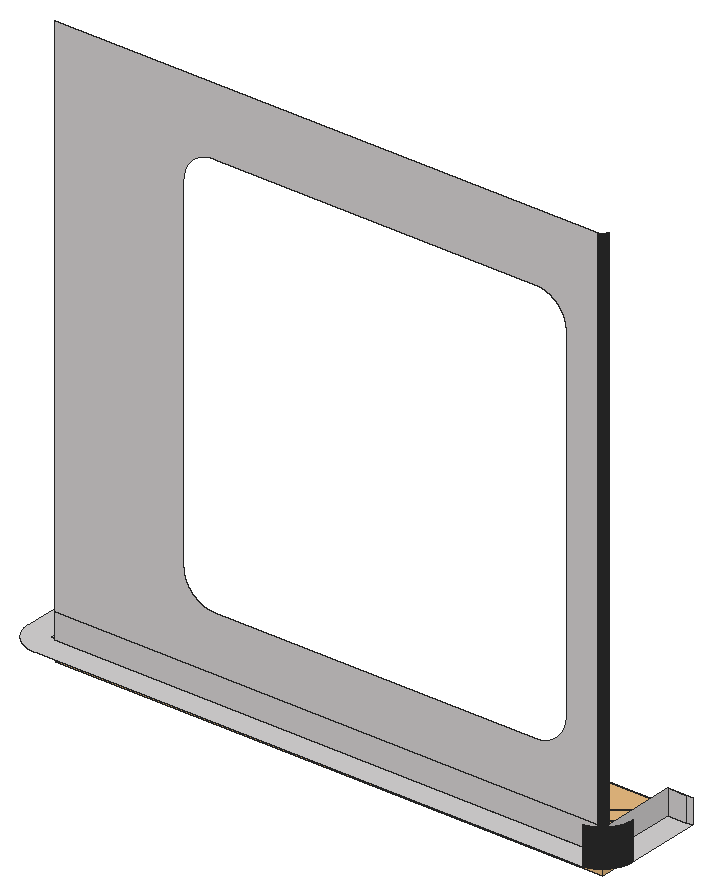
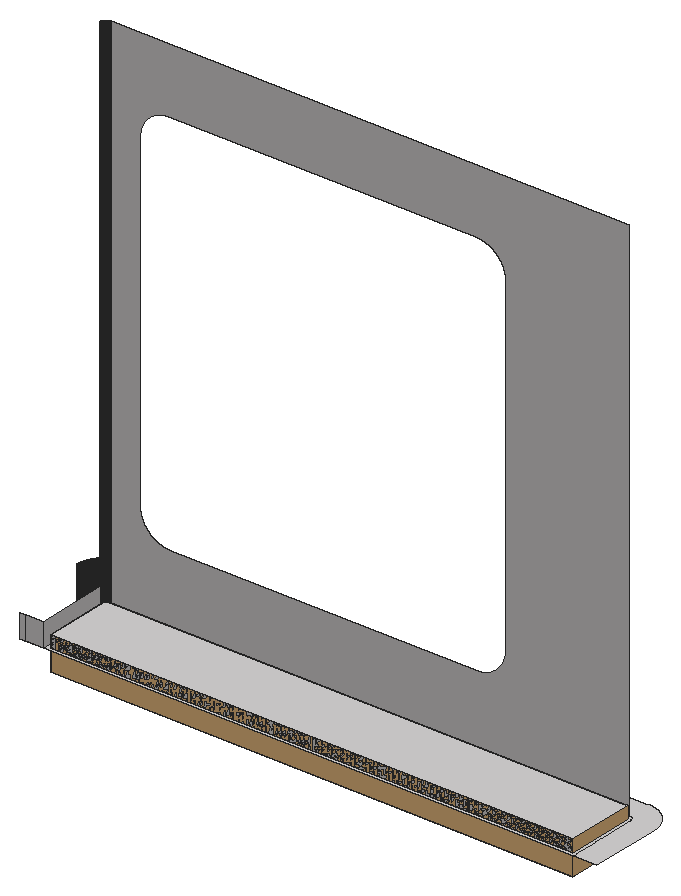
# SketchUp Ruby script. Lengths in inches.
U = 1.inch
M = Sketchup.active_model
def pt(a) = Geom::Point3d.new(a.map { |v| v * U })
def face(e, loops, mat)
  f = e.add_face(loops[0].map { |a| pt(a) })
  loops[1..].each { |l| e.add_face(l.map { |a| pt(a) }).erase! }
  f.material = f.back_material = mat if mat
  f
end
# faces: each face lists its corners as indices into pts; further lists are holes
def faces(e, pts, list, mat = nil) = list.each { |f| face(e, (f[0].is_a?(Array) ? f : [f]).map { |l| l.map { |i| pts[i] } }, mat) }
# xy, xz, yz: faces in a plane at the given z, y or x. An outline is a flat list of corners, or four numbers for a rectangle; further outlines are holes
def ring(l) = l.size == 4 ? [[l[0], l[1]], [l[2], l[1]], [l[2], l[3]], [l[0], l[3]]] : l.each_slice(2).to_a
def flat(e, list, mat, &to3) = list.each { |f| face(e, (f[0].is_a?(Array) ? f : [f]).map { |l| ring(l).map { |u, v| to3.(u, v) } }, mat) }
def xy(e, z, list, mat = nil) = flat(e, list, mat) { |x, y| [x, y, z] }
def xz(e, y, list, mat = nil) = flat(e, list, mat) { |x, z| [x, y, z] }
def yz(e, x, list, mat = nil) = flat(e, list, mat) { |y, z| [x, y, z] }
def lines(e, pts, list) = list.each { |a, b| e.add_line(pt(pts[a]), pt(pts[b])) }
# prism: a flat outline (further loops are holes) pulled along v
def prism(e, loops, v, mat = nil)
  f = face(e, loops, mat); d = Geom::Vector3d.new(v.map { |x| x * U })
  f.pushpull(f.normal.samedirection?(d) ? d.length : -d.length)
end
def box(e, o, s, mat = nil) = prism(e, [[o, [o[0] + s[0], o[1], o[2]], [o[0] + s[0], o[1] + s[1], o[2]], [o[0], o[1] + s[1], o[2]]]], [0, 0, s[2]], mat)
def at(x, y, z, deg = 0) = Geom::Transformation.translation(pt([x, y, z])) * Geom::Transformation.rotation(ORIGIN, Z_AXIS, deg.degrees)
def axes(o, x, y, z) = Geom::Transformation.new([*x, 0, *y, 0, *z, 0, *pt(o).to_a, 1])
def part(name) = M.definitions.add(name)
# library, detail: a bought-in or finely detailed component or shape, given as its bounding box
def library(name, o, s) = part(name).tap { |d| box(d.entities, o, s) }
def detail(e, o, s) = box(e.add_group.entities, o, s)
def put(e, d, t, mat = nil) = e.add_instance(d, t).tap { |i| i.material = mat if mat }
def group(e, t, mat = nil) = e.add_group.tap { |g| g.transformation = t; g.material = mat if mat }.entities
root = M.entities
M.materials.add("[Quartz Light Brown]").color = [215, 212, 212]
c1 = library("Group\#18",[0,0,-16.91],[266,35,16.91])
xy(root,114,[[216,143,215.804,143.001,215.607,143.005,215.411,143.012,215.215,143.021,215.019,143.032,214.823,143.046,214.627,143.063,214.432,143.082,214.237,143.104,214.042,143.128,213.848,143.155,213.653,143.185,213.46,143.217,213.266,143.251,213.074,143.288,212.881,143.328,212.69,143.37,212.498,143.414,212.308,143.462,212.118,143.511,211.928,143.563,211.74,143.618,211.552,143.675,211.365,143.734,211.178,143.796,210.993,143.86,210.808,143.927,210.624,143.996,210.442,144.068,210.26,144.142,210.079,144.218,209.899,144.297,209.72,144.378,209.542,144.461,209.366,144.547,209.19,144.635,209.016,144.725,208.843,144.818,208.671,144.913,208.5,145.01,208.331,145.109,208.163,145.21,207.996,145.314,207.83,145.42,207.666,145.528,207.504,145.638,207.343,145.75,207.183,145.865,207.025,145.981,206.869,146.1,206.714,146.22,206.56,146.343,206.408,146.467,206.258,146.594,206.11,146.722,205.963,146.853,205.818,146.985,205.675,147.119,205.533,147.255,205.393,147.393,205.255,147.533,205.119,147.675,204.985,147.818,204.853,147.963,204.722,148.11,204.594,148.258,204.467,148.408,204.343,148.56,204.22,148.714,204.1,148.869,203.981,149.025,203.865,149.183,203.75,149.343,203.638,149.504,203.528,149.666,203.42,149.83,203.314,149.996,203.21,150.163,203.109,150.331,203.01,150.5,202.913,150.671,202.818,150.843,202.725,151.016,202.635,151.19,202.547,151.366,202.461,151.542,202.378,151.72,202.297,151.899,202.218,152.079,202.142,152.26,202.068,152.442,201.996,152.624,201.927,152.808,201.86,152.993,201.796,153.178,201.734,153.365,201.675,153.552,201.618,153.74,201.563,153.928,201.511,154.118,201.462,154.308,201.414,154.498,201.37,154.69,201.328,154.881,201.288,155.074,201.251,155.266,201.217,155.46,201.185,155.653,201.155,155.848,201.128,156.042,201.104,156.237,201.082,156.432,201.063,156.627,201.046,156.823,201.032,157.019,201.021,157.215,201.012,157.411,201.005,157.607,201.001,157.804,201,158,201,194,213,194,213,157.961,213.001,157.921,213.003,157.881,213.01,157.764,213.021,157.647,213.037,157.53,213.058,157.414,213.083,157.299,213.113,157.185,213.147,157.073,213.186,156.962,213.229,156.852,213.276,156.744,213.327,156.638,213.382,156.535,213.442,156.433,213.505,156.334,213.573,156.237,213.644,156.143,213.718,156.052,213.796,155.965,213.878,155.88,213.963,155.798,214.051,155.72,214.142,155.645,214.235,155.574,214.332,155.507,214.431,155.443,214.532,155.384,214.636,155.328,214.742,155.277,214.85,155.229,214.959,155.186,215.07,155.148,215.183,155.113,215.297,155.084,215.412,155.058,215.528,155.037,215.644,155.021,215.761,155.01,215.879,155.002,215.921,155.001,215.961,155,480.082,155,480.196,155.006,480.311,155.015,480.425,155.029,480.538,155.048,480.651,155.071,480.762,155.098,480.873,155.129,480.982,155.164,481.09,155.204,481.196,155.248,481.3,155.295,481.403,155.347,481.503,155.403,481.601,155.462,481.697,155.525,481.791,155.592,481.881,155.662,481.969,155.736,482.054,155.813,482.137,155.893,482.216,155.976,482.291,156.063,482.364,156.152,482.433,156.244,482.498,156.338,482.56,156.435,482.618,156.534,482.672,156.635,482.722,156.738,482.768,156.843,482.811,156.95,482.849,157.058,482.883,157.168,482.912,157.279,482.9375,157.391,482.959,157.504,482.976,157.617,482.988,157.731,482.996,157.846,482.999,157.921,483,157.961,483,194,495,194,495,158,494.999,157.804,494.995,157.607,494.988,157.411,494.979,157.215,494.968,157.019,494.954,156.823,494.937,156.627,494.918,156.432,494.896,156.237,494.872,156.042,494.845,155.848,494.815,155.653,494.783,155.46,494.749,155.266,494.712,155.074,494.672,154.881,494.63,154.69,494.586,154.498,494.538,154.308,494.489,154.118,494.437,153.928,494.382,153.74,494.325,153.552,494.266,153.365,494.204,153.178,494.14,152.993,494.073,152.808,494.004,152.624,493.932,152.442,493.858,152.26,493.782,152.079,493.703,151.899,493.622,151.72,493.539,151.542,493.453,151.366,493.365,151.19,493.275,151.016,493.182,150.843,493.087,150.671,492.99,150.5,492.891,150.331,492.79,150.163,492.686,149.996,492.58,149.83,492.472,149.666,492.362,149.504,492.25,149.343,492.135,149.183,492.019,149.025,491.9,148.869,491.78,148.714,491.657,148.56,491.533,148.408,491.406,148.258,491.278,148.11,491.147,147.963,491.015,147.818,490.881,147.675,490.745,147.533,490.607,147.393,490.467,147.255,490.325,147.119,490.182,146.985,490.037,146.853,489.89,146.722,489.742,146.594,489.592,146.467,489.44,146.343,489.286,146.22,489.131,146.1,488.975,145.981,488.817,145.865,488.657,145.75,488.496,145.638,488.334,145.528,488.17,145.42,488.004,145.314,487.837,145.21,487.669,145.109,487.5,145.01,487.329,144.913,487.157,144.818,486.984,144.725,486.81,144.635,486.634,144.547,486.458,144.461,486.28,144.378,486.101,144.297,485.921,144.218,485.74,144.142,485.558,144.068,485.376,143.996,485.192,143.927,485.007,143.86,484.822,143.796,484.635,143.734,484.448,143.675,484.26,143.618,484.072,143.563,483.882,143.511,483.692,143.462,483.502,143.414,483.31,143.37,483.119,143.328,482.926,143.288,482.734,143.251,482.54,143.217,482.347,143.185,482.152,143.155,481.958,143.128,481.763,143.104,481.568,143.082,481.373,143.063,481.177,143.046,480.981,143.032,480.785,143.021,480.589,143.012,480.393,143.005,480.196,143.001,480,143],[[216,155,215.882,155.002,215.765,155.009,215.648,155.021,215.531,155.037,215.415,155.058,215.3,155.083,215.186,155.113,215.073,155.147,214.962,155.185,214.852,155.228,214.744,155.276,214.638,155.327,214.534,155.383,214.433,155.442,214.333,155.506,214.237,155.573,214.143,155.644,214.052,155.719,213.964,155.797,213.879,155.879,213.797,155.964,213.719,156.052,213.644,156.143,213.573,156.237,213.506,156.333,213.442,156.433,213.383,156.534,213.327,156.638,213.276,156.744,213.229,156.852,213.186,156.962,213.147,157.073,213.113,157.186,213.083,157.3,213.058,157.415,213.037,157.531,213.021,157.647,213.009,157.765,213.002,157.882,213,158,213,194,483,194,482.999,157.921,482.994,157.808,482.984,157.694,482.971,157.581,482.953,157.469,482.93,157.357,482.904,157.246,482.873,157.136,482.838,157.028,482.8,156.921,482.757,156.815,482.71,156.712,482.659,156.61,482.604,156.51,482.546,156.412,482.484,156.317,482.418,156.224,482.349,156.133,482.276,156.045,482.201,155.96,482.122,155.878,482.04,155.799,481.955,155.723,481.867,155.651,481.776,155.582,481.683,155.516,481.588,155.454,481.49,155.395,481.39,155.341,481.288,155.29,481.184,155.243,481.079,155.2,480.972,155.161,480.863,155.126,480.754,155.095,480.643,155.069,480.531,155.046,480.419,155.028,480.306,155.015,480.192,155.005,480.079,155],[480.026,156.999,480.064,157.001,480.102,157.004,480.139,157.009,480.177,157.015,480.214,157.022,480.251,157.031,480.288,157.041,480.324,157.053,480.36,157.066,480.395,157.08,480.429,157.096,480.463,157.113,480.497,157.131,480.561,157.171,480.592,157.193,480.622,157.216,480.651,157.24,480.68,157.266,480.707,157.292,480.733,157.319,480.759,157.348,480.783,157.377,480.806,157.407,480.828,157.438,480.849,157.47,480.868,157.503,480.886,157.536,480.903,157.57,480.919,157.605,480.933,157.64,480.946,157.675,480.958,157.712,480.968,157.748,480.977,157.785,480.984,157.822,480.99,157.86,480.995,157.898,480.998,157.935,481,157.973,481,192,215,192,215,158,215.001,157.961,215.003,157.922,215.007,157.882,215.012,157.844,215.019,157.805,215.028,157.767,215.038,157.729,215.049,157.691,215.062,157.654,215.076,157.617,215.092,157.581,215.109,157.546,215.128,157.511,215.148,157.478,215.169,157.444,215.191,157.412,215.215,157.381,215.24,157.351,215.266,157.321,215.293,157.293,215.321,157.266,215.351,157.24,215.381,157.215,215.412,157.191,215.478,157.147,215.546,157.109,215.582,157.092,215.617,157.076,215.654,157.062,215.691,157.049,215.729,157.038,215.767,157.028,215.805,157.019,215.844,157.012,215.883,157.007,215.922,157.003,215.961,157.001,216,157]]],"[Quartz Light Brown]")
xy(root,120,[[480.026,156.999,216,157,215.961,157.001,215.922,157.003,215.883,157.007,215.844,157.012,215.805,157.019,215.767,157.028,215.729,157.038,215.691,157.049,215.654,157.062,215.617,157.076,215.582,157.092,215.546,157.109,215.478,157.147,215.412,157.191,215.381,157.215,215.351,157.24,215.321,157.266,215.293,157.293,215.266,157.321,215.24,157.351,215.215,157.381,215.191,157.412,215.169,157.444,215.148,157.478,215.128,157.511,215.109,157.546,215.092,157.581,215.076,157.617,215.062,157.654,215.049,157.691,215.038,157.729,215.028,157.767,215.019,157.805,215.012,157.844,215.007,157.882,215.003,157.922,215.001,157.961,215,158,215,192,481,192,481,157.973,480.998,157.935,480.995,157.898,480.99,157.86,480.984,157.822,480.977,157.785,480.968,157.748,480.958,157.712,480.946,157.675,480.933,157.64,480.919,157.605,480.903,157.57,480.886,157.536,480.868,157.503,480.849,157.47,480.828,157.438,480.806,157.407,480.783,157.377,480.759,157.348,480.733,157.319,480.707,157.292,480.68,157.266,480.651,157.24,480.622,157.216,480.592,157.193,480.561,157.171,480.497,157.131,480.463,157.113,480.429,157.096,480.395,157.08,480.36,157.066,480.324,157.053,480.288,157.041,480.251,157.031,480.214,157.022,480.177,157.015,480.139,157.009,480.102,157.004,480.064,157.001]],"[Quartz Light Brown]")
xz(root,155,[[216,114,480.079,126],[480.079,114,480.082,126]],"[Quartz Light Brown]")
xz(root,192,[[215,114,481,120]],"[Quartz Light Brown]")
xz(root,194,[[483,114,492,126],[483,114,495,126]],"[Quartz Light Brown]")
yz(root,481,[[157.973,114,192,120]],"[Quartz Light Brown]")
p = [[482.152,143.155,132],[482.152,143.155,114],[482.347,143.185,114],[482.347,143.185,132],[482.54,143.217,114],[482.54,143.217,132],
  [482.734,143.251,114],[482.734,143.251,132],[482.926,143.288,114],[482.926,143.288,132],[483.119,143.328,114],[483.119,143.328,132],
  [483.31,143.37,114],[483.31,143.37,132],[483.502,143.414,114],[483.502,143.414,132],[483.692,143.462,114],[483.692,143.462,132],
  [483.882,143.511,114],[483.882,143.511,132],[484.072,143.563,114],[484.072,143.563,132],[484.26,143.618,114],[484.26,143.618,132],
  [484.448,143.675,114],[484.448,143.675,132],[484.635,143.734,114],[484.635,143.734,132],[484.822,143.796,114],[484.822,143.796,132],
  [485.007,143.86,114],[485.007,143.86,132],[485.192,143.927,114],[485.192,143.927,132],[485.376,143.996,114],[485.376,143.996,132],
  [485.558,144.068,114],[485.558,144.068,132],[485.74,144.142,114],[485.74,144.142,132],[485.921,144.218,114],[485.921,144.218,132],
  [486.101,144.297,114],[486.101,144.297,132],[486.28,144.378,114],[486.28,144.378,132],[486.458,144.461,114],[486.458,144.461,132],
  [486.634,144.547,114],[486.634,144.547,132],[486.81,144.635,114],[486.81,144.635,132],[486.984,144.725,114],[486.984,144.725,132],
  [487.157,144.818,114],[487.157,144.818,132],[487.329,144.913,114],[487.329,144.913,132],[487.5,145.01,114],[487.5,145.01,132],
  [487.669,145.109,114],[487.669,145.109,132],[487.837,145.21,114],[487.837,145.21,132],[488.004,145.314,114],[488.004,145.314,132],
  [488.17,145.42,114],[488.17,145.42,132],[488.334,145.528,114],[488.334,145.528,132],[488.496,145.638,114],[488.496,145.638,132],
  [488.657,145.75,114],[488.657,145.75,132],[488.817,145.865,114],[488.817,145.865,132],[488.975,145.981,114],[488.975,145.981,132],
  [489.131,146.1,114],[489.131,146.1,132],[489.286,146.22,114],[489.286,146.22,132],[489.44,146.343,114],[489.44,146.343,132],
  [489.592,146.467,114],[489.592,146.467,132],[489.742,146.594,114],[489.742,146.594,132],[489.89,146.722,114],[489.89,146.722,132],
  [490.037,146.853,114],[490.037,146.853,132],[490.182,146.985,114],[490.182,146.985,132],[490.325,147.119,114],[490.325,147.119,132],
  [490.467,147.255,114],[490.467,147.255,132],[490.607,147.393,114],[490.607,147.393,132],[490.745,147.533,114],[490.745,147.533,132],
  [490.881,147.675,114],[490.881,147.675,132],[491.015,147.818,114],[491.015,147.818,132],[491.147,147.963,114],[491.147,147.963,132],
  [491.278,148.11,114],[491.278,148.11,132],[491.406,148.258,114],[491.406,148.258,132],[491.533,148.408,114],[491.533,148.408,132],
  [491.657,148.56,114],[491.657,148.56,132],[491.78,148.714,114],[491.78,148.714,132],[491.9,148.869,114],[491.9,148.869,132],
  [492.019,149.025,114],[492.019,149.025,132],[492.135,149.183,114],[492.135,149.183,132],[492.25,149.343,114],[492.25,149.343,132],
  [492.362,149.504,114],[492.362,149.504,132],[492.472,149.666,114],[492.472,149.666,132],[492.58,149.83,114],[492.58,149.83,132],
  [492.686,149.996,114],[492.686,149.996,132],[492.79,150.163,114],[492.79,150.163,132],[492.891,150.331,114],[492.891,150.331,132],
  [492.99,150.5,114],[492.99,150.5,132],[493.087,150.671,114],[493.087,150.671,132],[493.182,150.843,114],[493.182,150.843,132],
  [493.275,151.016,114],[493.275,151.016,132],[493.365,151.19,114],[493.365,151.19,132],[493.453,151.366,114],[493.453,151.366,132],
  [493.539,151.542,114],[493.539,151.542,132],[493.622,151.72,114],[493.622,151.72,132],[493.703,151.899,114],[493.703,151.899,132],
  [493.782,152.079,114],[493.782,152.079,132],[493.858,152.26,114],[493.858,152.26,132],[493.932,152.442,114],[493.932,152.442,132],
  [494.004,152.624,114],[494.004,152.624,132],[494.073,152.808,114],[494.073,152.808,132],[494.14,152.993,114],[494.14,152.993,132],
  [494.204,153.178,114],[494.204,153.178,132],[494.266,153.365,114],[494.266,153.365,132],[494.325,153.552,114],[494.325,153.552,132],
  [494.382,153.74,114],[494.382,153.74,132],[494.437,153.928,114],[494.437,153.928,132],[494.489,154.118,114],[494.489,154.118,132],
  [494.538,154.308,114],[494.538,154.308,132],[494.586,154.498,114],[494.586,154.498,132],[494.63,154.69,114],[494.63,154.69,132],
  [494.672,154.881,114],[494.672,154.881,132],[494.712,155.074,114],[494.712,155.074,132],[216,155,126],[215.882,155.002,126],
  [215.882,155.002,114],[216,155,114],[215.961,155,114],[215.961,155,384],[216,155,384],[480.079,155.001,384],
  [480.079,155,126],[480.079,155,114],[216,155,114],[215.996,155,114],[464.979,155,336.785],[464.968,155,336.981],
  [464.954,155,337.177],[464.937,155,337.373],[464.918,155,337.568],[464.896,155,337.763],[464.872,155,337.958],[464.845,155,338.152],
  [464.815,155,338.347],[464.783,155,338.54],[464.749,155,338.734],[464.712,155,338.926],[464.672,155,339.119],[464.63,155,339.31],
  [464.586,155,339.502],[464.538,155,339.692],[464.489,155,339.882],[464.437,155,340.072],[464.382,155,340.26],[464.325,155,340.448],
  [464.266,155,340.635],[464.204,155,340.822],[464.14,155,341.007],[464.073,155,341.192],[464.004,155,341.376],[463.932,155,341.558],
  [463.858,155,341.74],[463.782,155,341.921],[463.703,155,342.101],[463.622,155,342.28],[463.539,155,342.458],[463.453,155,342.634],
  [463.365,155,342.81],[463.275,155,342.984],[463.182,155,343.157],[463.087,155,343.329],[462.99,155,343.5],[462.891,155,343.669],
  [462.79,155,343.837],[462.686,155,344.004],[462.58,155,344.17],[462.472,155,344.334],[462.362,155,344.496],[462.25,155,344.657],
  [462.135,155,344.817],[462.019,155,344.975],[461.9,155,345.131],[461.78,155,345.286],[461.657,155,345.44],[461.533,155,345.592],
  [461.406,155,345.742],[461.278,155,345.89],[461.147,155,346.037],[461.015,155,346.182],[460.881,155,346.325],[460.745,155,346.467],
  [460.607,155,346.607],[460.467,155,346.745],[460.325,155,346.881],[460.182,155,347.015],[460.037,155,347.147],[459.89,155,347.278],
  [459.742,155,347.406],[459.592,155,347.533],[459.44,155,347.657],[459.286,155,347.78],[459.131,155,347.9],[458.975,155,348.019],
  [458.817,155,348.135],[458.657,155,348.25],[458.496,155,348.362],[458.334,155,348.472],[458.17,155,348.58],[458.004,155,348.686],
  [457.837,155,348.79],[457.669,155,348.891],[457.5,155,348.99],[457.329,155,349.087],[457.157,155,349.182],[456.984,155,349.275],
  [456.81,155,349.365],[456.634,155,349.453],[456.458,155,349.539],[456.28,155,349.622],[456.101,155,349.703],[455.921,155,349.782],
  [455.74,155,349.858],[455.558,155,349.932],[455.376,155,350.004],[455.192,155,350.073],[455.007,155,350.14],[454.822,155,350.204],
  [454.635,155,350.266],[454.448,155,350.325],[454.26,155,350.382],[454.072,155,350.437],[453.882,155,350.489],[453.692,155,350.538],
  [453.502,155,350.586],[453.31,155,350.63],[453.119,155,350.672],[452.926,155,350.712],[452.734,155,350.749],[452.54,155,350.783],
  [452.347,155,350.815],[452.152,155,350.845],[451.958,155,350.872],[451.763,155,350.896],[451.568,155,350.918],[451.373,155,350.937],
  [451.177,155,350.954],[450.981,155,350.968],[450.785,155,350.979],[450.589,155,350.988],[450.393,155,350.995],[450.196,155,350.999],
  [450,155,351],[293.5,155,351],[293.304,155,350.999],[293.107,155,350.995],[292.911,155,350.988],[292.715,155,350.979],
  [292.519,155,350.968],[292.323,155,350.954],[292.127,155,350.937],[291.932,155,350.918],[291.737,155,350.896],[291.542,155,350.872],
  [291.348,155,350.845],[291.153,155,350.815],[290.96,155,350.783],[290.766,155,350.749],[290.574,155,350.712],[290.381,155,350.672],
  [290.19,155,350.63],[289.998,155,350.586],[289.808,155,350.538],[289.618,155,350.489],[289.428,155,350.437],[289.24,155,350.382],
  [289.052,155,350.325],[288.865,155,350.266],[288.678,155,350.204],[288.493,155,350.14],[288.308,155,350.073],[288.124,155,350.004],
  [287.942,155,349.932],[287.76,155,349.858],[287.579,155,349.782],[287.399,155,349.703],[287.22,155,349.622],[287.042,155,349.539],
  [286.866,155,349.453],[286.69,155,349.365],[286.516,155,349.275],[286.343,155,349.182],[286.171,155,349.087],[286,155,348.99],
  [285.831,155,348.891],[285.663,155,348.79],[285.496,155,348.686],[285.33,155,348.58],[285.166,155,348.472],[285.004,155,348.362],
  [284.843,155,348.25],[284.683,155,348.135],[284.525,155,348.019],[284.369,155,347.9],[284.214,155,347.78],[284.06,155,347.657],
  [283.908,155,347.533],[283.758,155,347.406],[283.61,155,347.278],[283.463,155,347.147],[283.318,155,347.015],[283.175,155,346.881],
  [283.033,155,346.745],[282.893,155,346.607],[282.755,155,346.467],[282.619,155,346.325],[282.485,155,346.182],[282.353,155,346.037],
  [282.222,155,345.89],[282.094,155,345.742],[281.967,155,345.592],[281.843,155,345.44],[281.72,155,345.286],[281.6,155,345.131],
  [281.481,155,344.975],[281.365,155,344.817],[281.25,155,344.657],[281.138,155,344.496],[281.028,155,344.334],[280.92,155,344.17],
  [280.814,155,344.004],[280.71,155,343.837],[280.609,155,343.669],[280.51,155,343.5],[280.413,155,343.329],[280.318,155,343.157],
  [280.225,155,342.984],[280.135,155,342.81],[280.047,155,342.634],[279.961,155,342.458],[279.878,155,342.28],[279.797,155,342.101],
  [279.718,155,341.921],[279.642,155,341.74],[279.568,155,341.558],[279.496,155,341.376],[279.427,155,341.192],[279.36,155,341.007],
  [279.296,155,340.822],[279.234,155,340.635],[279.175,155,340.448],[279.118,155,340.26],[279.063,155,340.072],[279.011,155,339.882],
  [278.962,155,339.692],[278.914,155,339.502],[278.87,155,339.31],[278.828,155,339.119],[278.788,155,338.926],[278.751,155,338.734],
  [278.717,155,338.54],[278.685,155,338.347],[278.655,155,338.152],[278.628,155,337.958],[278.604,155,337.763],[278.582,155,337.568],
  [278.563,155,337.373],[278.546,155,337.177],[278.532,155,336.981],[278.521,155,336.785],[278.512,155,336.589],[278.505,155,336.393],
  [278.501,155,336.196],[278.5,155,336],[278.5,155,168],[278.501,155,167.804],[278.505,155,167.607],[278.512,155,167.411],
  [278.521,155,167.215],[278.532,155,167.019],[278.546,155,166.823],[278.563,155,166.627],[278.582,155,166.432],[278.604,155,166.237],
  [278.628,155,166.042],[278.655,155,165.848],[278.685,155,165.653],[278.717,155,165.46],[278.751,155,165.266],[278.788,155,165.074],
  [278.828,155,164.881],[278.87,155,164.69],[278.914,155,164.498],[278.962,155,164.308],[279.011,155,164.118],[279.063,155,163.928],
  [279.118,155,163.74],[279.175,155,163.552],[279.234,155,163.365],[279.296,155,163.178],[279.36,155,162.993],[279.427,155,162.808],
  [279.496,155,162.624],[279.568,155,162.442],[279.642,155,162.26],[279.718,155,162.079],[279.797,155,161.899],[279.878,155,161.72],
  [279.961,155,161.542],[280.047,155,161.366],[280.135,155,161.19],[280.225,155,161.016],[280.318,155,160.843],[280.413,155,160.671],
  [280.51,155,160.5],[280.609,155,160.331],[280.71,155,160.163],[280.814,155,159.996],[280.92,155,159.83],[281.028,155,159.666],
  [281.138,155,159.504],[281.25,155,159.343],[281.365,155,159.183],[281.481,155,159.025],[281.6,155,158.869],[281.72,155,158.714],
  [281.843,155,158.56],[281.967,155,158.408],[282.094,155,158.258],[282.222,155,158.11],[282.353,155,157.963],[282.485,155,157.818],
  [282.619,155,157.675],[282.755,155,157.533],[282.893,155,157.393],[283.033,155,157.255],[283.175,155,157.119],[283.318,155,156.985],
  [283.463,155,156.853],[283.61,155,156.722],[283.758,155,156.594],[283.908,155,156.467],[284.06,155,156.343],[284.214,155,156.22],
  [284.369,155,156.1],[284.525,155,155.981],[284.683,155,155.865],[284.843,155,155.75],[285.004,155,155.638],[285.166,155,155.528],
  [285.33,155,155.42],[285.496,155,155.314],[285.663,155,155.21],[285.831,155,155.109],[286,155,155.01],[286.171,155,154.913],
  [286.343,155,154.818],[286.516,155,154.725],[286.69,155,154.635],[286.866,155,154.547],[287.042,155,154.461],[287.22,155,154.378],
  [287.399,155,154.297],[287.579,155,154.218],[287.76,155,154.142],[287.942,155,154.068],[288.124,155,153.996],[288.308,155,153.927],
  [288.493,155,153.86],[288.678,155,153.796],[288.865,155,153.734],[289.052,155,153.675],[289.24,155,153.618],[289.428,155,153.563],
  [289.618,155,153.511],[289.808,155,153.462],[289.998,155,153.414],[290.19,155,153.37],[290.381,155,153.328],[290.574,155,153.288],
  [290.766,155,153.251],[290.96,155,153.217],[291.153,155,153.185],[291.348,155,153.155],[291.542,155,153.128],[291.737,155,153.104],
  [291.932,155,153.082],[292.127,155,153.063],[292.323,155,153.046],[292.519,155,153.032],[292.715,155,153.021],[292.911,155,153.012],
  [293.107,155,153.005],[293.304,155,153.001],[293.5,155,153],[450,155,153],[450.196,155,153.001],[450.393,155,153.005],
  [450.589,155,153.012],[450.785,155,153.021],[450.981,155,153.032],[451.177,155,153.046],[451.373,155,153.063],[451.568,155,153.082],
  [451.763,155,153.104],[451.958,155,153.128],[452.152,155,153.155],[452.347,155,153.185],[452.54,155,153.217],[452.734,155,153.251],
  [452.926,155,153.288],[453.119,155,153.328],[453.31,155,153.37],[453.502,155,153.414],[453.692,155,153.462],[453.882,155,153.511],
  [454.072,155,153.563],[454.26,155,153.618],[454.448,155,153.675],[454.635,155,153.734],[454.822,155,153.796],[455.007,155,153.86],
  [455.192,155,153.927],[455.376,155,153.996],[455.558,155,154.068],[455.74,155,154.142],[455.921,155,154.218],[456.101,155,154.297],
  [456.28,155,154.378],[456.458,155,154.461],[456.634,155,154.547],[456.81,155,154.635],[456.984,155,154.725],[457.157,155,154.818],
  [457.329,155,154.913],[457.5,155,155.01],[457.669,155,155.109],[457.837,155,155.21],[458.004,155,155.314],[458.17,155,155.42],
  [458.334,155,155.528],[458.496,155,155.638],[458.657,155,155.75],[458.817,155,155.865],[458.975,155,155.981],[459.131,155,156.1],
  [459.286,155,156.22],[459.44,155,156.343],[459.592,155,156.467],[459.742,155,156.594],[459.89,155,156.722],[460.037,155,156.853],
  [460.182,155,156.985],[460.325,155,157.119],[460.467,155,157.255],[460.607,155,157.393],[460.745,155,157.533],[460.881,155,157.675],
  [461.015,155,157.818],[461.147,155,157.963],[461.278,155,158.11],[461.406,155,158.258],[461.533,155,158.408],[461.657,155,158.56],
  [461.78,155,158.714],[461.9,155,158.869],[462.019,155,159.025],[462.135,155,159.183],[462.25,155,159.343],[462.362,155,159.504],
  [462.472,155,159.666],[462.58,155,159.83],[462.686,155,159.996],[462.79,155,160.163],[462.891,155,160.331],[462.99,155,160.5],
  [463.087,155,160.671],[463.182,155,160.843],[463.275,155,161.016],[463.365,155,161.19],[463.453,155,161.366],[463.539,155,161.542],
  [463.622,155,161.72],[463.703,155,161.899],[463.782,155,162.079],[463.858,155,162.26],[463.932,155,162.442],[464.004,155,162.624],
  [464.073,155,162.808],[464.14,155,162.993],[464.204,155,163.178],[464.266,155,163.365],[464.325,155,163.552],[464.382,155,163.74],
  [464.437,155,163.928],[464.489,155,164.118],[464.538,155,164.308],[464.586,155,164.498],[464.63,155,164.69],[464.672,155,164.881],
  [464.712,155,165.074],[464.749,155,165.266],[464.783,155,165.46],[464.815,155,165.653],[464.845,155,165.848],[464.872,155,166.042],
  [464.896,155,166.237],[464.918,155,166.432],[464.937,155,166.627],[464.954,155,166.823],[464.968,155,167.019],[464.979,155,167.215],
  [464.988,155,167.411],[464.995,155,167.607],[464.999,155,167.804],[465,155,168],[465,155,336],[464.999,155,336.196],
  [464.995,155,336.393],[464.988,155,336.589],[480.192,155.005,126],[480.079,155,126],[480.079,155,114],[480.192,155.005,114],
  [480.082,155,114],[480.196,155.006,114],[480.196,155.006,126],[480.196,155.006,384],[480.157,155.004,384],[480.118,155.002,384],
  [480.082,155,384],[480.082,155,126],[480.306,155.015,126],[480.306,155.015,114],[480.311,155.015,114],[480.311,155.016,126],
  [480.311,155.015,384],[480.275,155.013,384],[480.235,155.009,384],[480.419,155.028,126],[480.419,155.028,114],[480.425,155.029,114],
  [480.425,155.03,126],[480.425,155.029,384],[480.392,155.026,384],[480.353,155.021,384],[480.314,155.016,384],[480.531,155.046,126],
  [480.531,155.046,114],[480.538,155.048,114],[480.538,155.048,126],[480.538,155.048,384],[480.508,155.043,384],[480.469,155.037,384],
  [480.43,155.031,384],[480.643,155.069,126],[480.643,155.069,114],[480.651,155.071,114],[480.651,155.071,126],[480.651,155.071,384],
  [480.624,155.066,384],[480.585,155.058,384],[480.547,155.05,384],[480.754,155.095,126],[480.754,155.095,114],[480.762,155.098,114],
  [480.762,155.098,126],[480.762,155.098,384],[480.738,155.092,384],[480.7,155.083,384],[480.662,155.074,384],[480.863,155.126,126],
  [480.863,155.126,114],[480.873,155.129,114],[480.873,155.129,126],[480.873,155.129,384],[480.852,155.124,384],[480.814,155.113,384],
  [480.776,155.102,384],[480.972,155.161,126],[480.972,155.161,114],[480.982,155.164,114],[480.982,155.165,126],[480.982,155.164,384],
  [480.964,155.159,384],[480.927,155.147,384],[480.89,155.135,384],[494.749,155.266,114],[494.749,155.266,132],[481.079,155.2,126],
  [481.079,155.2,114],[481.09,155.204,114],[481.089,155.204,126],[481.09,155.204,384],[481.075,155.199,384],[481.038,155.185,384],
  [481.001,155.172,384],[481.184,155.243,126],[481.184,155.243,114],[481.196,155.248,114],[481.196,155.248,126],[481.196,155.248,384],
  [481.184,155.244,384],[481.148,155.228,384],[481.112,155.214,384],[481.288,155.29,126],[481.288,155.29,114],[481.3,155.295,114],
  [481.3,155.296,126],[481.3,155.295,384],[481.292,155.292,384],[481.256,155.276,384],[481.22,155.259,384],[481.39,155.341,126],
  [481.39,155.341,114],[481.403,155.347,114],[481.402,155.348,126],[481.403,155.347,384],[481.397,155.345,384],[481.362,155.327,384],
  [481.327,155.309,384],[481.49,155.395,126],[481.49,155.395,114],[481.503,155.403,114],[481.503,155.403,126],[481.503,155.403,384],
  [481.5,155.402,384],[481.466,155.383,384],[481.431,155.364,384],[494.783,155.46,114],[494.783,155.46,132],[481.588,155.454,126],
  [481.588,155.454,114],[481.601,155.462,114],[481.601,155.463,126],[481.601,155.463,384],[481.567,155.442,384],[481.534,155.422,384],
  [481.683,155.516,126],[481.683,155.516,114],[481.697,155.525,114],[481.697,155.526,126],[481.697,155.525,384],[481.667,155.506,384],
  [481.634,155.484,384],[481.776,155.582,126],[481.776,155.582,114],[481.791,155.592,114],[481.79,155.592,126],[481.791,155.592,384],
  [481.763,155.573,384],[481.731,155.55,384],[481.699,155.528,384],[494.815,155.653,114],[494.815,155.653,132],[481.867,155.651,126],
  [481.867,155.651,114],[481.881,155.662,114],[481.881,155.663,126],[481.881,155.662,384],[481.857,155.644,384],[481.826,155.62,384],
  [481.795,155.596,384],[481.955,155.723,126],[481.955,155.723,114],[481.969,155.736,114],[481.969,155.736,126],[481.969,155.736,384],
  [481.948,155.719,384],[481.918,155.693,384],[481.888,155.669,384],[482.04,155.799,126],[482.04,155.799,114],[482.054,155.813,114],
  [482.054,155.813,126],[482.054,155.813,384],[482.036,155.797,384],[482.007,155.771,384],[481.978,155.744,384],[494.845,155.848,114],
  [494.845,155.848,132],[482.122,155.878,126],[482.122,155.878,114],[482.137,155.893,114],[482.136,155.893,126],[482.137,155.893,384],
  [482.121,155.879,384],[482.093,155.851,384],[482.065,155.824,384],[494.872,156.042,114],[494.872,156.042,132],[482.201,155.96,126],
  [482.201,155.96,114],[482.216,155.976,114],[482.215,155.977,126],[482.216,155.976,384],[482.203,155.964,384],[482.176,155.935,384],
  [482.149,155.907,384],[482.276,156.045,126],[482.276,156.045,114],[482.291,156.063,114],[482.291,156.063,126],[482.291,156.063,384],
  [482.281,156.052,384],[482.256,156.022,384],[482.229,155.993,384],[482.349,156.133,126],[482.349,156.133,114],[494.896,156.237,114],
  [494.896,156.237,132],[482.418,156.224,126],[482.418,156.224,114],[482.364,156.152,114],[482.364,156.152,126],[482.364,156.152,384],
  [482.356,156.143,384],[482.333,156.114,384],[482.331,156.112,384],[482.329,156.109,384],[482.307,156.082,384],[482.484,156.317,126],
  [482.484,156.317,114],[482.433,156.244,114],[482.432,156.244,126],[482.433,156.244,384],[482.427,156.237,384],[482.406,156.209,384],
  [482.404,156.205,384],[482.397,156.196,384],[482.38,156.174,384],[482.498,156.338,114],[482.498,156.338,126],[482.498,156.338,384],
  [482.494,156.333,384],[482.476,156.306,384],[482.472,156.301,384],[482.46,156.283,384],[482.45,156.269,384],[494.918,156.432,114],
  [494.918,156.432,132],[482.546,156.412,126],[482.546,156.412,114],[482.56,156.435,114],[482.56,156.435,126],[482.56,156.435,384],
  [482.558,156.433,384],[482.541,156.405,384],[482.537,156.399,384],[482.516,156.366,384],[482.604,156.51,126],[482.604,156.51,114],
  [482.618,156.534,114],[482.617,156.534,126],[482.617,156.534,384],[482.602,156.507,384],[482.598,156.5,384],[482.578,156.466,384],
  [482.576,156.462,384],[494.937,156.627,114],[494.937,156.627,132],[482.659,156.61,126],[482.659,156.61,114],[482.672,156.635,114],
  [482.672,156.635,126],[482.672,156.635,384],[482.659,156.61,384],[482.655,156.603,384],[482.636,156.569,384],[482.632,156.561,384],
  [482.71,156.712,126],[482.71,156.712,114],[482.722,156.738,114],[482.722,156.738,126],[482.722,156.738,384],[482.711,156.716,384],
  [482.708,156.708,384],[482.691,156.673,384],[482.684,156.661,384],[482.673,156.638,384],[494.954,156.823,114],[494.954,156.823,132],
  [482.757,156.815,126],[482.757,156.815,114],[482.768,156.843,114],[482.768,156.843,126],[482.768,156.843,384],[482.76,156.823,384],
  [482.756,156.816,384],[482.741,156.78,384],[482.732,156.762,384],[482.724,156.744,384],[482.8,156.921,126],[482.8,156.921,114],
  [482.811,156.95,114],[482.81,156.95,126],[482.811,156.95,384],[482.804,156.932,384],[482.801,156.925,384],[482.786,156.888,384],
  [482.777,156.864,384],[482.772,156.852,384],[494.968,157.019,114],[494.968,157.019,132],[482.838,157.028,126],[482.838,157.028,114],
  [215.961,157.001,114],[215.922,157.003,114],[215.922,157.003,120],[215.961,157.001,120],[216,157,114],[216,157,120],
  [480.026,156.999,114],[480.026,156.999,120],[480.064,157.001,114],[480.064,157.001,120],[480.102,157.004,114],[480.102,157.004,120],
  [480.139,157.009,114],[480.139,157.009,120],[480.177,157.015,114],[480.177,157.015,120],[480.214,157.022,114],[480.214,157.022,120],
  [480.251,157.031,114],[480.251,157.031,120],[480.288,157.041,114],[480.288,157.041,120],[480.324,157.053,114],[480.324,157.053,120],
  [482.873,157.136,126],[482.873,157.136,114],[482.849,157.058,114],[482.849,157.058,126],[482.849,157.058,384],[482.843,157.043,384],
  [482.841,157.036,384],[482.828,156.999,384],[482.816,156.967,384],[482.815,156.962,384],[494.979,157.215,114],[494.979,157.215,132],
  [480.36,157.066,114],[480.36,157.066,120],[480.395,157.08,114],[480.395,157.08,120],[480.429,157.096,114],[480.429,157.096,120],
  [480.463,157.113,114],[480.463,157.113,120],[480.497,157.131,114],[480.497,157.131,120],[480.529,157.151,114],[480.529,157.151,120],
  [482.883,157.168,114],[482.882,157.168,126],[482.883,157.168,384],[482.878,157.155,384],[482.876,157.148,384],[482.865,157.11,384],
  [482.853,157.073,384],[482.853,157.071,384],[482.904,157.246,126],[482.904,157.246,114],[480.561,157.171,114],[480.561,157.171,120],
  [480.592,157.193,114],[480.592,157.193,120],[480.622,157.216,114],[480.622,157.216,120],[480.651,157.24,114],[480.651,157.24,120],
  [480.68,157.266,114],[480.68,157.266,120],[482.93,157.357,126],[482.93,157.357,114],[482.912,157.279,114],[482.912,157.279,126],
  [482.912,157.279,384],[482.909,157.268,384],[482.908,157.262,384],[482.898,157.224,384],[482.887,157.186,384],[482.886,157.18,384],
  [494.988,157.411,114],[494.988,157.411,132],[480.707,157.292,114],[480.707,157.292,120],[480.733,157.319,114],[480.733,157.319,120],
  [480.759,157.348,114],[480.759,157.348,120],[480.783,157.377,114],[480.783,157.377,120],[482.9375,157.391,114],[482.9375,157.391,126],
  [482.9375,157.391,384],[482.936,157.382,384],[482.934,157.376,384],[482.926,157.338,384],[482.917,157.3,384],[482.915,157.29,384],
  [480.806,157.407,114],[480.806,157.407,120],[480.828,157.438,114],[480.828,157.438,120],[480.849,157.47,114],[480.849,157.47,120],
  [482.953,157.469,126],[482.953,157.469,114],[482.959,157.504,114],[482.959,157.504,126],[482.959,157.504,384],[482.958,157.497,384],
  [482.957,157.492,384],[482.95,157.453,384],[482.942,157.415,384],[482.94,157.401,384],[494.995,157.607,114],[494.995,157.607,132],
  [480.868,157.503,114],[480.868,157.503,120],[480.886,157.536,114],[480.886,157.536,120],[480.903,157.57,114],[480.903,157.57,120],
  [482.971,157.581,126],[482.971,157.581,114],[482.976,157.617,114],[482.976,157.617,126],[482.976,157.617,384],[482.975,157.613,384],
  [482.974,157.608,384],[482.969,157.57,384],[482.963,157.531,384],[482.96,157.512,384],[480.919,157.605,114],[480.919,157.605,120],
  [480.933,157.64,114],[480.933,157.64,120],[480.946,157.675,114],[480.946,157.675,120],[482.984,157.694,126],[482.984,157.694,114],
  [482.988,157.731,114],[482.988,157.731,126],[482.988,157.731,384],[482.988,157.729,384],[482.987,157.725,384],[482.984,157.686,384],
  [482.979,157.647,384],[482.976,157.623,384],[494.999,157.804,114],[494.999,157.804,132],[480.958,157.712,114],[480.958,157.712,120],
  [480.968,157.748,114],[480.968,157.748,120],[480.977,157.785,114],[480.977,157.785,120],[482.994,157.808,126],[482.994,157.808,114],
  [482.996,157.846,114],[482.996,157.846,126],[482.996,157.846,384],[482.996,157.843,384],[482.994,157.804,384],[482.991,157.765,384],
  [482.988,157.735,384],[480.984,157.822,114],[480.984,157.822,120],[480.99,157.86,114],[480.99,157.86,120],[482.999,157.921,126],
  [482.999,157.921,114],[482.999,157.921,114],[482.999,157.921,126],[482.999,157.921,384],[482.998,157.882,384],[495,158,114],
  [495,158,132],[480.995,157.898,114],[480.995,157.898,120],[480.998,157.935,114],[480.998,157.935,120],[481,157.973,114],
  [481,157.973,120],[483,194,114],[483,194,126],[483,157.961,384],[483,157.961,114],[483,155,120],
  [483,155,126]]
faces(root,p,[[0,1,2,3],[3,2,4,5],[5,4,6,7],[7,6,8,9],[9,8,10,11],[11,10,12,13],[13,12,14,15],[15,14,16,17],
  [17,16,18,19],[19,18,20,21],[21,20,22,23],[23,22,24,25],[25,24,26,27],[27,26,28,29],[29,28,30,31],[31,30,32,33],
  [33,32,34,35],[35,34,36,37],[37,36,38,39],[39,38,40,41],[41,40,42,43],[43,42,44,45],[45,44,46,47],[47,46,48,49],
  [49,48,50,51],[51,50,52,53],[53,52,54,55],[55,54,56,57],[57,56,58,59],[59,58,60,61],[61,60,62,63],[63,62,64,65],
  [65,64,66,67],[67,66,68,69],[69,68,70,71],[71,70,72,73],[73,72,74,75],[75,74,76,77],[77,76,78,79],[79,78,80,81],
  [81,80,82,83],[83,82,84,85],[85,84,86,87],[87,86,88,89],[89,88,90,91],[91,90,92,93],[93,92,94,95],[95,94,96,97],
  [97,96,98,99],[99,98,100,101],[101,100,102,103],[103,102,104,105],[105,104,106,107],[107,106,108,109],[109,108,110,111],[111,110,112,113],
  [113,112,114,115],[115,114,116,117],[117,116,118,119],[119,118,120,121],[121,120,122,123],[123,122,124,125],[125,124,126,127],[127,126,128,129],
  [129,128,130,131],[131,130,132,133],[133,132,134,135],[135,134,136,137],[137,136,138,139],[139,138,140,141],[141,140,142,143],[143,142,144,145],
  [145,144,146,147],[147,146,148,149],[149,148,150,151],[151,150,152,153],[153,152,154,155],[155,154,156,157],[157,156,158,159],[159,158,160,161],
  [161,160,162,163],[163,162,164,165],[165,164,166,167],[167,166,168,169],[169,168,170,171],[171,170,172,173],[173,172,174,175],[175,174,176,177],
  [177,176,178,179],[179,178,180,181],[181,180,182,183],[183,182,184,185],[185,184,186,187],[187,186,188,189],[190,191,192,193],[[194,195,196,197,198,199,200,201],[202,203,204,205,206,207,208,209,210,211,212,213,214,215,216,217,218,219,220,221,222,223,224,225,226,227,228,229,230,231,232,233,234,235,236,237,238,239,240,241,242,243,244,245,246,247,248,249,250,251,252,253,254,255,256,257,258,259,260,261,262,263,264,265,266,267,268,269,270,271,272,273,274,275,276,277,278,279,280,281,282,283,284,285,286,287,288,289,290,291,292,293,294,295,296,297,298,299,300,301,302,303,304,305,306,307,308,309,310,311,312,313,314,315,316,317,318,319,320,321,322,323,324,325,326,327,328,329,330,331,332,333,334,335,336,337,338,339,340,341,342,343,344,345,346,347,348,349,350,351,352,353,354,355,356,357,358,359,360,361,362,363,364,365,366,367,368,369,370,371,372,373,374,375,376,377,378,379,380,381,382,383,384,385,386,387,388,389,390,391,392,393,394,395,396,397,398,399,400,401,402,403,404,405,406,407,408,409,410,411,412,413,414,415,416,417,418,419,420,421,422,423,424,425,426,427,428,429,430,431,432,433,434,435,436,437,438,439,440,441,442,443,444,445,446,447,448,449,450,451,452,453,454,455,456,457,458,459,460,461,462,463,464,465,466,467,468,469,470,471,472,473,474,475,476,477,478,479,480,481,482,483,484,485,486,487,488,489,490,491,492,493,494,495,496,497,498,499,500,501,502,503,504,505,506,507,508,509,510,511,512,513,514,515,516,517,518,519,520,521,522,523,524,525,526,527,528,529,530,531,532,533,534,535,536,537,538,539,540,541,542,543,544,545,546,547,548,549,550,551,552,553,554,555,556,557,558,559,560,561,562,563,564,565,566,567,568,569,570,571,572,573,574,575,576,577,578,579,580,581,582,583,584,585,586,587,588,589,590,591,592,593,594,595,596,597,598,599,600,601,602,603,604,605,606,607,608,609,610,611,612,613,614,615,616,617,618,619,620,621,622,623,624,625,626,627,628,629,630,631,632,633,634,635,636,637,638,639,640,641,642,643,644,645,646,647,648,649,650,651,652,653,654,655,656,657,658,659,660,661,662,663,664,665,666,667,668,669,670,671,672,673,674,675,676,677,678,679,680,681,682,683,684,685]],
  [686,687,688,689],[690,691,692,693,694,695,696,697],[698,686,689,699],[691,700,701,702,703,704,693,692],[705,698,699,706],[700,707,708,709,710,711,712,702,701],[713,705,706,714],[707,715,716,717,718,719,720,709,708],
  [721,713,714,722],[715,723,724,725,726,727,728,717,716],[729,721,722,730],[723,731,732,733,734,735,736,725,724],[737,729,730,738],[731,739,740,741,742,743,744,733,732],[745,737,738,746],[739,747,748,749,750,751,752,741,740],
  [189,188,753,754],[755,745,746,756],[747,757,758,759,760,761,762,749,748],[763,755,756,764],[757,765,766,767,768,769,770,759,758],[771,763,764,772],[765,773,774,775,776,777,778,767,766],[779,771,772,780],
  [773,781,782,783,784,785,786,775,774],[787,779,780,788],[781,789,790,791,792,793,794,783,782],[754,753,795,796],[797,787,788,798],[789,799,800,801,802,803,791,790],[804,797,798,805],[799,806,807,808,809,810,801,800],
  [811,804,805,812],[806,813,814,815,816,817,818,808,807],[796,795,819,820],[821,811,812,822],[813,823,824,825,826,827,828,815,814],[829,821,822,830],[823,831,832,833,834,835,836,825,824],[837,829,830,838],
  [831,839,840,841,842,843,844,833,832],[820,819,845,846],[847,837,838,848],[839,849,850,851,852,853,854,841,840],[846,845,855,856],[857,847,848,858],[849,859,860,861,862,863,864,851,850],[865,857,858,866],
  [859,867,868,869,870,871,872,861,860],[873,865,866,874],[856,855,875,876],[877,873,874,878],[867,879,880,881,882,883,884,885,886,869,868],[887,877,878,888],[879,889,890,891,892,893,894,895,896,881,880],[889,897,898,899,900,901,902,903,904,891,890],
  [876,875,905,906],[907,887,888,908],[897,909,910,911,912,913,914,915,899,898],[916,907,908,917],[909,918,919,920,921,922,923,924,911,910],[906,905,925,926],[927,916,917,928],[918,929,930,931,932,933,934,935,920,919],
  [936,927,928,937],[929,938,939,940,941,942,943,944,945,931,930],[926,925,946,947],[948,936,937,949],[938,950,951,952,953,954,955,956,957,940,939],[958,948,949,959],[950,960,961,962,963,964,965,966,967,952,951],[947,946,968,969],
  [970,958,959,971],[972,973,974,975],[976,972,975,977],[978,976,977,979],[980,978,979,981],[982,980,981,983],[984,982,983,985],[986,984,985,987],
  [988,986,987,989],[990,988,989,991],[992,990,991,993],[994,992,993,995],[996,970,971,997],[960,998,999,1000,1001,1002,1003,1004,1005,962,961],[969,968,1006,1007],[1008,994,995,1009],
  [1010,1008,1009,1011],[1012,1010,1011,1013],[1014,1012,1013,1015],[1016,1014,1015,1017],[1018,1016,1017,1019],[998,1020,1021,1022,1023,1024,1025,1026,1027,1000,999],[1028,996,997,1029],[1030,1018,1019,1031],
  [1032,1030,1031,1033],[1034,1032,1033,1035],[1036,1034,1035,1037],[1038,1036,1037,1039],[1040,1028,1029,1041],[1020,1042,1043,1044,1045,1046,1047,1048,1049,1022,1021],[1007,1006,1050,1051],[1052,1038,1039,1053],
  [1054,1052,1053,1055],[1056,1054,1055,1057],[1058,1056,1057,1059],[1042,1060,1061,1062,1063,1064,1065,1066,1067,1044,1043],[1068,1058,1059,1069],[1070,1068,1069,1071],[1072,1070,1071,1073],[1074,1040,1041,1075],
  [1060,1076,1077,1078,1079,1080,1081,1082,1083,1062,1061],[1051,1050,1084,1085],[1086,1072,1073,1087],[1088,1086,1087,1089],[1090,1088,1089,1091],[1092,1074,1075,1093],[1076,1094,1095,1096,1097,1098,1099,1100,1101,1078,1077],[1102,1090,1091,1103],
  [1104,1102,1103,1105],[1106,1104,1105,1107],[1108,1092,1093,1109],[1094,1110,1111,1112,1113,1114,1115,1116,1117,1096,1095],[1085,1084,1118,1119],[1120,1106,1107,1121],[1122,1120,1121,1123],[1124,1122,1123,1125],
  [1126,1108,1109,1127],[1110,1128,1129,1130,1131,1132,1133,1134,1112,1111],[1135,1124,1125,1136],[1137,1135,1136,1138],[1139,1126,1127,1140],[1128,1141,1142,1143,1144,1130,1129],[1119,1118,1145,1146],[1147,1137,1138,1148],
  [1149,1147,1148,1150],[1151,1149,1150,1152],[1139,1140,1153,1154],[1143,1155,1156,1141,1142]],"[Quartz Light Brown]")
lines(root,p,[[1157,1158]])
put(root,c1,at(215,157,120),"[Quartz Light Brown]")
